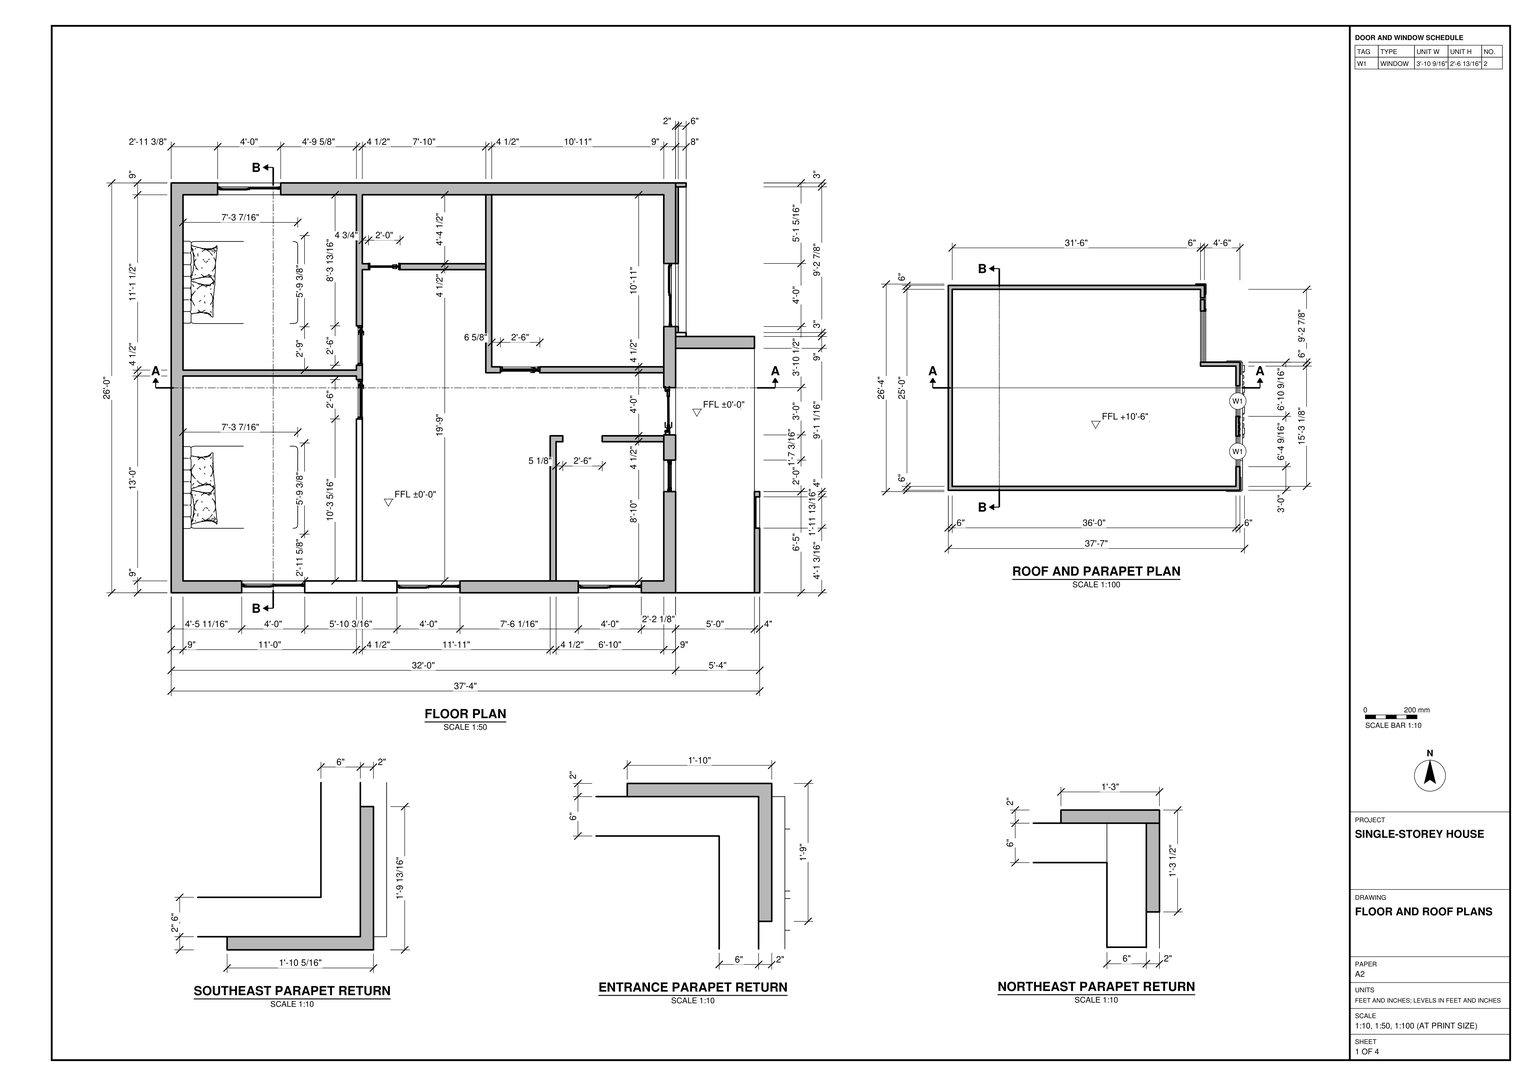
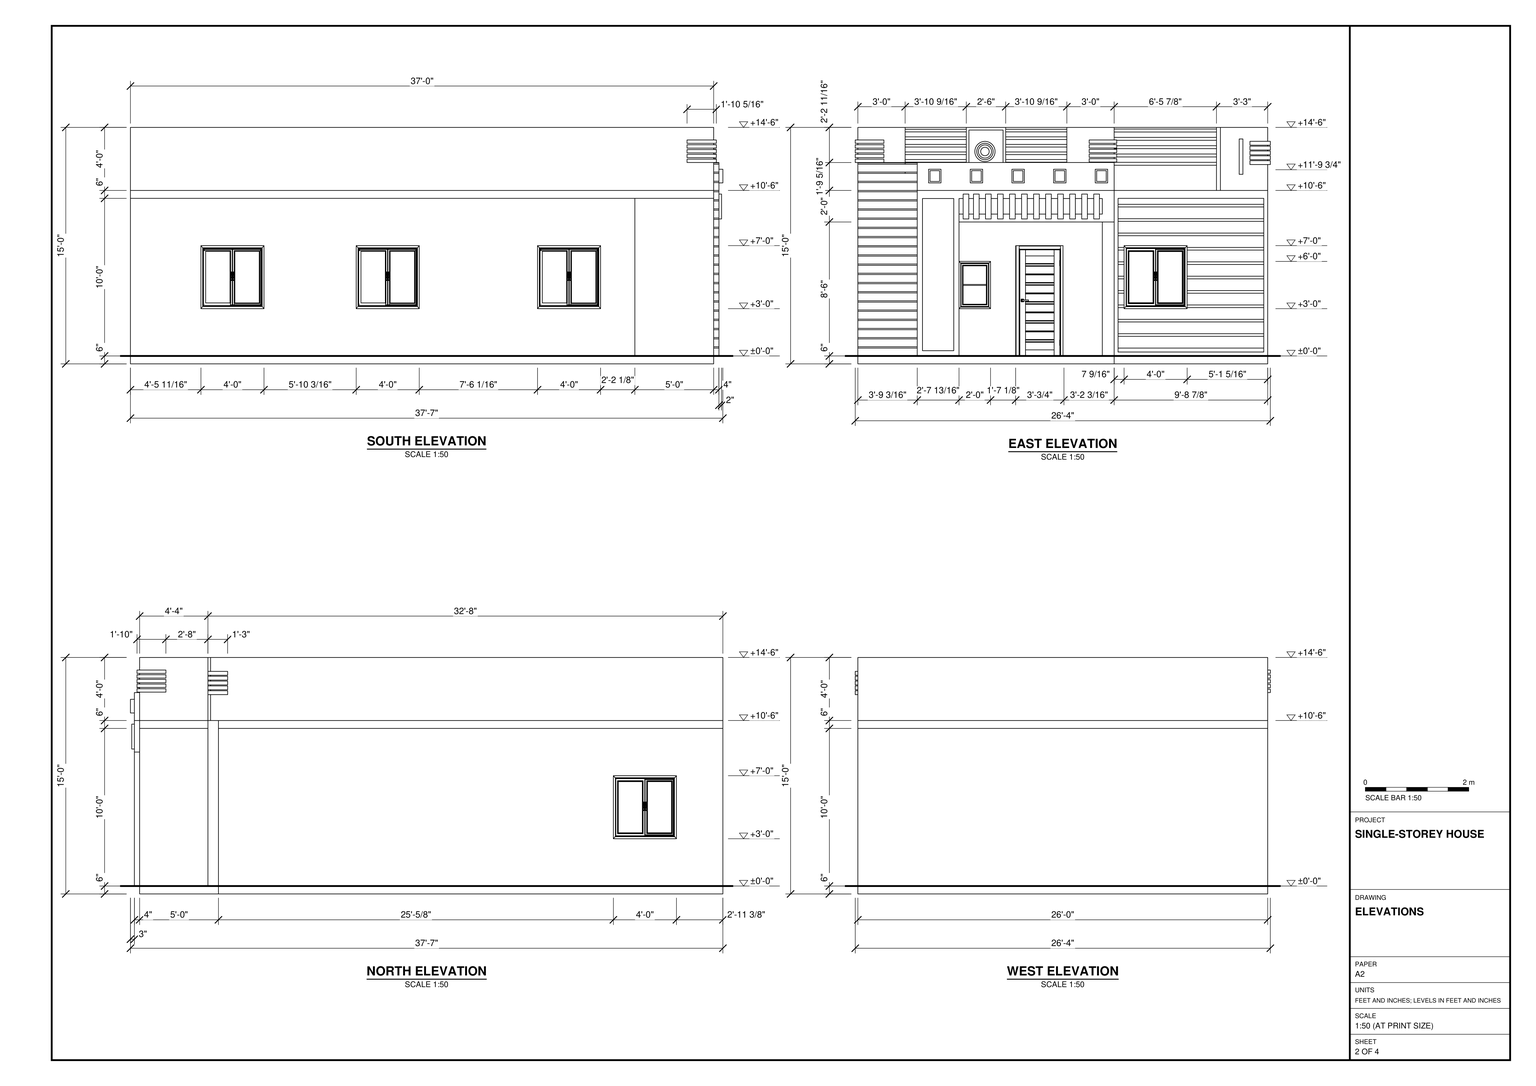
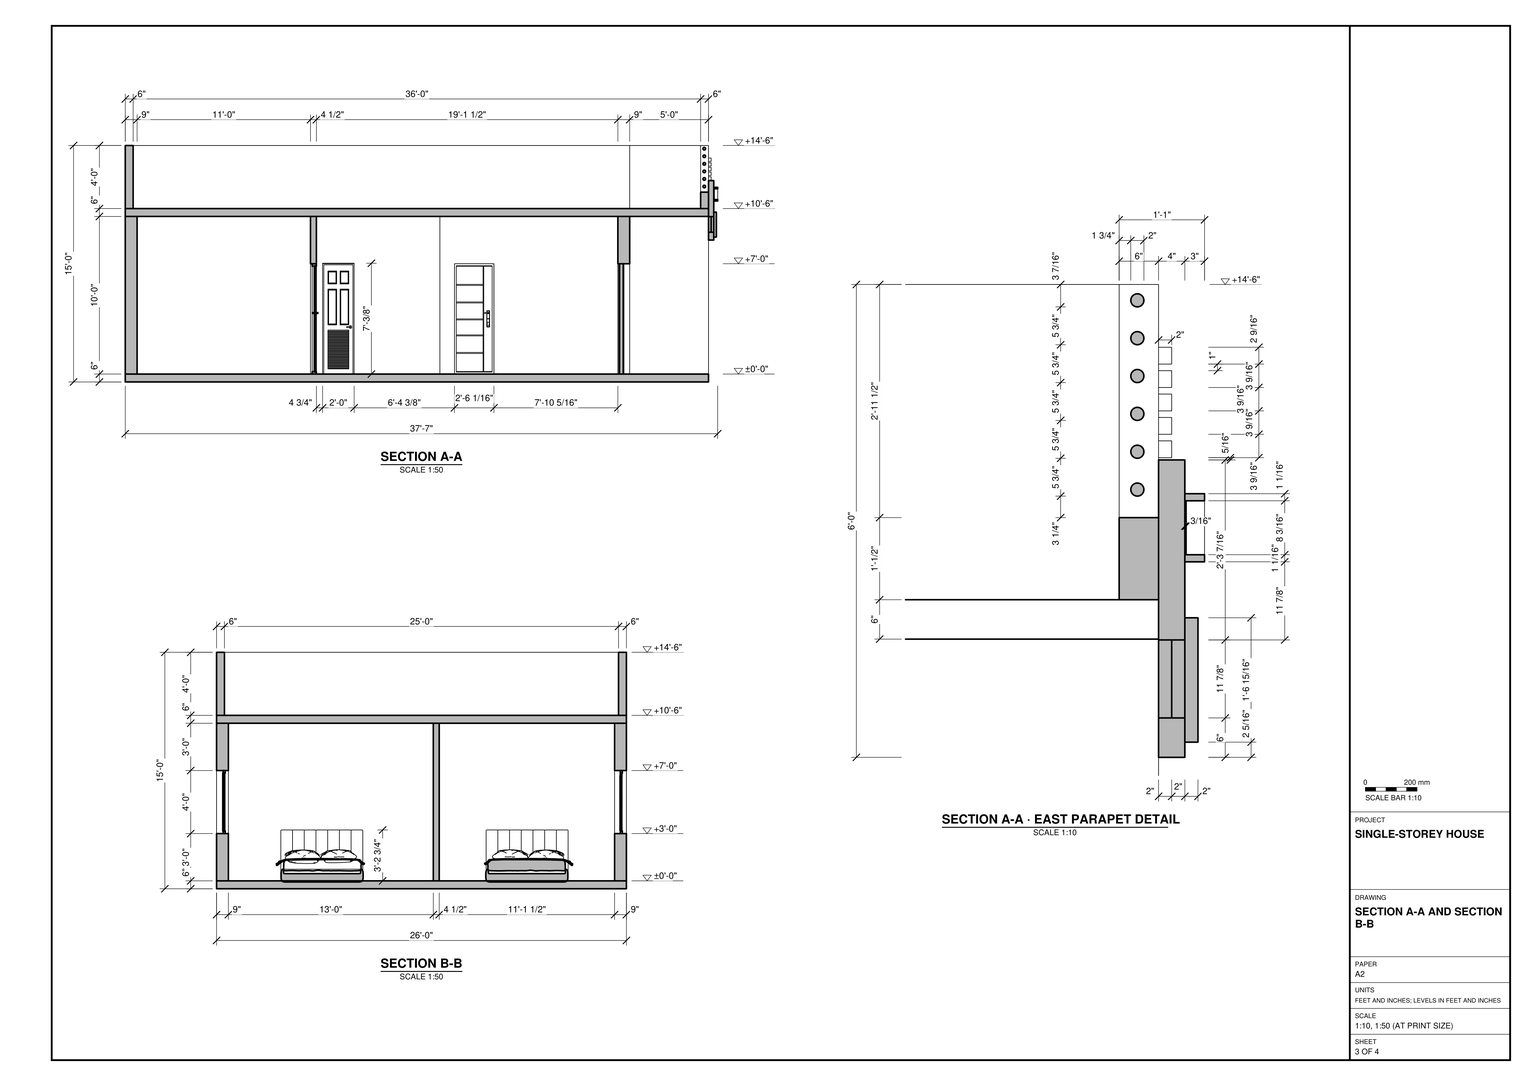
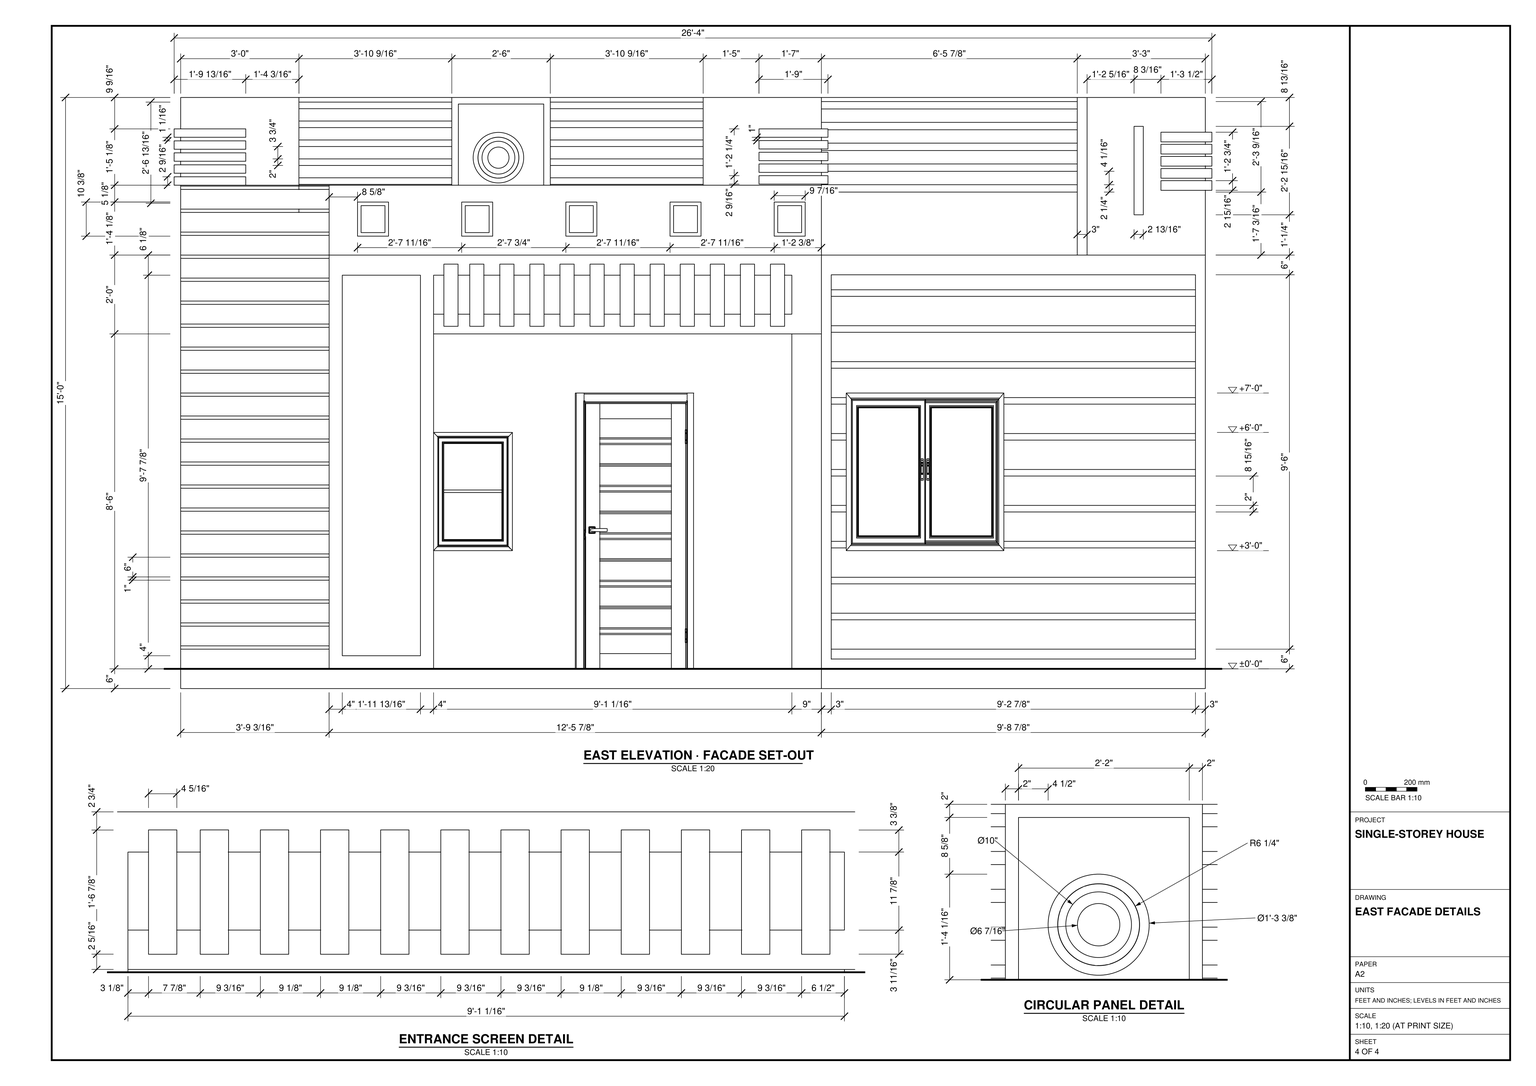
Build the single-storey house in SketchUp using task_files/diagram_01.pdf. Work in feet and inches. Set the finished ground floor at ±0'-0" and model the full exterior, including the slab edges and parapet returns, to an overall size of 37'-7" east to west by 26'-4" north to south by 15'-0" high.

Lay out the main exterior walls at 9" thick and the interior partitions at 4 1/2" thick where indicated. Follow the plan for the two west bedrooms, central circulation space, remaining rooms and covered east entrance. Fit the doors and framed windows in the positions shown. Place a bed against the west wall of each bedroom, matching its footprint in plan and its headboard in section.

Model the floor and flat roof slabs. Set the roof surface at +10'-6" and carry the parapet around the stepped roof outline to +14'-6". Use the east elevation and parapet details to shape the horizontal bands, entrance surround and corner returns; keep the other elevations plain where shown. Decor and loose items may be any suitable library components.

Keep walls, slabs, roof and individual furniture or joinery pieces in separate groups or components, and use components for repeated parts. Save one SketchUp model as output_files/single_storey_house_with_a_recessed_east_entrance.skp.

# SketchUp Ruby script. Lengths in inches.
U = 1.inch
M = Sketchup.active_model
def pt(a) = Geom::Point3d.new(a.map { |v| v * U })
def face(e, loops, mat)
  f = e.add_face(loops[0].map { |a| pt(a) })
  loops[1..].each { |l| e.add_face(l.map { |a| pt(a) }).erase! }
  f.material = f.back_material = mat if mat
  f
end
# faces: each face lists its corners as indices into pts; further lists are holes
def faces(e, pts, list, mat = nil) = list.each { |f| face(e, (f[0].is_a?(Array) ? f : [f]).map { |l| l.map { |i| pts[i] } }, mat) }
# xy, xz, yz: faces in a plane at the given z, y or x. An outline is a flat list of corners, or four numbers for a rectangle; further outlines are holes
def ring(l) = l.size == 4 ? [[l[0], l[1]], [l[2], l[1]], [l[2], l[3]], [l[0], l[3]]] : l.each_slice(2).to_a
def flat(e, list, mat, &to3) = list.each { |f| face(e, (f[0].is_a?(Array) ? f : [f]).map { |l| ring(l).map { |u, v| to3.(u, v) } }, mat) }
def xy(e, z, list, mat = nil) = flat(e, list, mat) { |x, y| [x, y, z] }
def xz(e, y, list, mat = nil) = flat(e, list, mat) { |x, z| [x, y, z] }
def yz(e, x, list, mat = nil) = flat(e, list, mat) { |y, z| [x, y, z] }
def lines(e, pts, list) = list.each { |a, b| e.add_line(pt(pts[a]), pt(pts[b])) }
# prism: a flat outline (further loops are holes) pulled along v
def prism(e, loops, v, mat = nil)
  f = face(e, loops, mat); d = Geom::Vector3d.new(v.map { |x| x * U })
  f.pushpull(f.normal.samedirection?(d) ? d.length : -d.length)
end
def box(e, o, s, mat = nil) = prism(e, [[o, [o[0] + s[0], o[1], o[2]], [o[0] + s[0], o[1] + s[1], o[2]], [o[0], o[1] + s[1], o[2]]]], [0, 0, s[2]], mat)
def at(x, y, z, deg = 0) = Geom::Transformation.translation(pt([x, y, z])) * Geom::Transformation.rotation(ORIGIN, Z_AXIS, deg.degrees)
def axes(o, x, y, z) = Geom::Transformation.new([*x, 0, *y, 0, *z, 0, *pt(o).to_a, 1])
def part(name) = M.definitions.add(name)
# library, detail: a bought-in or finely detailed component or shape, given as its bounding box
def library(name, o, s) = part(name).tap { |d| box(d.entities, o, s) }
def detail(e, o, s) = box(e.add_group.entities, o, s)
def put(e, d, t, mat = nil) = e.add_instance(d, t).tap { |i| i.material = mat if mat }
def group(e, t, mat = nil) = e.add_group.tap { |g| g.transformation = t; g.material = mat if mat }.entities
root = M.entities
M.materials.add("[0003_DeepPink]").color = [255, 20, 147]
M.materials.add("[0005_LightPink]").color = [255, 182, 193]
M.materials.add("[0057_DarkKhaki]").color = [189, 183, 107]
M.materials.add("[0080_DarkCyan]").color = [0, 139, 139]
M.materials.add("[0100_SteelBlue]").color = [70, 130, 180]
M.materials.add("[0109_DarkSlateBlue]").color = [72, 61, 139]
M.materials.add("[0110_LightSlateGray]").color = [119, 136, 153]
M.materials.add("[0127_Magenta]").color = [255, 0, 255]
M.materials.add("[Color A08]").color = [51, 51, 51]
M.materials.add("[Color B07]").color = [153, 38, 0]
M.materials.add("[Color F06]").color = [102, 204, 0]
M.materials.add("[Color H03]").color = [101, 255, 255]
M.materials.add("[Color J07]").color = [76, 0, 153]
M.materials.add("[Color M03]3").color = [132, 147, 124]
M.materials.add("[Color M06]1").color = [61, 61, 61]
M.materials.add("[Field Rectangle Tile]").color = [196, 189, 179]
M.materials.add("[Metal_Corrogated_Shiny]13").color = [12, 12, 12]
M.materials.add("[Metal_Corrogated_Shiny]6").color = [193, 193, 193]
M.materials.add("[Translucent Glass Gray]").color = [128, 128, 128]
c1 = part("Doorknob_Lever_Utility")
xy(c1.entities,0,[[-0.625,-1.08,-1.25,0,-0.625,1.08,0.625,1.08,1.25,0,0.625,-1.08]])
xy(c1.entities,0.25,[[[-0.625,-1.08,0.625,-1.08,1.25,0,0.625,1.08,-0.625,1.08,-1.25,0],[-0.19,-0.33,-0.38,0,-0.19,0.33,0.19,0.33,0.38,0,0.19,-0.33]]])
xy(c1.entities,1.9375,[[-0.19,-0.33,0.19,-0.33,0.38,0,0.19,0.33,-0.19,0.33]])
xz(c1.entities,-1.08,[[-0.625,0,0.625,0.25]])
xz(c1.entities,-0.33,[[-0.19,0.25,0.19,0.25,0.19,1.9375,-0.19,1.9375,-1.49,1.92,-2.79,1.8,-2.75,1.55,-1.48,1.67,-0.19,1.6875]])
xz(c1.entities,0.33,[[-0.19,0.25,-0.19,1.6875,-1.48,1.67,-2.75,1.55,-2.79,1.8,-1.49,1.92,-0.19,1.9375,0.19,1.9375,0.19,0.25]])
xz(c1.entities,1.08,[[-0.625,0,0.625,0.25]])
p = [[-1.25,0,0],[-0.625,-1.08,0],[-0.625,-1.08,0.25],[-1.25,0,0.25],[0.625,-1.08,0],[1.25,0,0],
  [1.25,0,0.25],[0.625,-1.08,0.25],[-0.625,1.08,0],[-0.625,1.08,0.25],[0.625,1.08,0],[0.625,1.08,0.25],
  [-0.19,-0.33,0.25],[-0.19,-0.33,1.6875],[-0.38,0,1.69],[-0.38,0,0.25],[0.19,-0.33,0.25],[0.38,0,0.25],
  [0.38,0,1.9375],[0.19,-0.33,1.9375],[-0.19,0.33,1.6875],[-0.19,0.33,0.25],[0.19,0.33,0.25],[0.19,0.33,1.9375],
  [-4.02,-0.21,1.32],[-2.75,-0.33,1.55],[-4.07,-0.21,1.5625],[-4.02,0.21,1.32],[-2.75,0.33,1.55],[-4.07,0.21,1.5625],
  [-2.79,-0.33,1.8],[-1.48,0.33,1.67],[-1.48,-0.33,1.67],[-2.79,0.33,1.8],[-1.49,-0.33,1.92],[-1.49,0.33,1.92],
  [-0.19,-0.33,1.9375],[-0.19,0.33,1.9375]]
faces(c1.entities,p,[[0,1,2,3],[4,5,6,7],[8,0,3,9],[5,10,11,6],[12,13,14,15],[16,17,18,19],[15,14,20,21],[17,22,23,18],
  [24,25,26],[27,28,25,24],[24,26,29,27],[27,29,28],[30,26,25],[28,31,32,25],[33,28,29],[26,30,33,29],
  [13,32,31,20,14],[33,30,34,35],[36,37,35,34]])
c2 = part("群組\#205")
prism(c2.entities,[[[6.69,3.9375,84.37],[6.69,3.9375,0],[6.69,5.12,0],[6.69,5.12,83.1875],[6.69,34.25,83.1875],[6.69,34.25,0],[6.69,35.43,0],[6.69,35.43,84.37]]],[-7.3,0,0])
c3 = part("群組\#206")
xy(c3.entities,0,[[0,0,1.18,29.13]])
xy(c3.entities,3.95,[[-0.12,4.16,0,24.97],[1.18,4.16,1.3,24.97]])
xy(c3.entities,4.07,[[-0.12,4.28,1.3,24.85]])
xy(c3.entities,33.36,[[-0.12,4.28,1.3,24.85]])
xy(c3.entities,33.48,[[-0.12,4.16,0,24.97],[1.18,4.16,1.3,24.97]])
xy(c3.entities,83.1875,[[0,0,1.18,29.13]])
xz(c3.entities,0,[[0,0,1.18,83.1875]])
xz(c3.entities,4.16,[[-0.12,3.95,0,33.48],[1.18,3.95,1.3,33.48]])
xz(c3.entities,4.28,[[-0.12,4.07,1.3,33.36]])
xz(c3.entities,24.85,[[-0.12,4.07,1.3,33.36]])
xz(c3.entities,24.97,[[-0.12,3.95,0,33.48],[1.18,3.95,1.3,33.48]])
xz(c3.entities,29.13,[[0,0,1.18,83.1875]])
yz(c3.entities,-0.12,[[[4.16,3.95,24.97,33.48],[4.28,4.07,24.85,33.36]]])
yz(c3.entities,0,[[[0,0,29.13,83.1875],[4.16,3.95,24.97,33.48],[16.3,37.41,24.97,64.69],[4.16,37.41,12.83,64.69],[16.3,68.62,24.97,78.46],[4.16,68.62,12.83,78.46]],[4.86,38.2,12.14,63.9],[16.99,38.2,24.28,63.9],[4.86,69.41,12.14,77.68],[16.99,69.41,24.28,77.68]])
yz(c3.entities,0.12,[[[4.27,37.53,12.73,64.57],[4.75,38.08,12.24,64.02]],[[16.41,37.53,24.87,64.57],[16.89,38.08,24.38,64.02]],[[4.27,68.74,12.73,78.35],[4.75,69.29,12.24,77.8]],[[16.41,68.74,24.87,78.35],[16.89,69.29,24.38,77.8]]])
yz(c3.entities,1.0625,[[[4.27,37.53,12.73,64.57],[4.75,38.08,12.24,64.02]],[[16.41,37.53,24.87,64.57],[16.89,38.08,24.38,64.02]],[[4.27,68.74,12.73,78.35],[4.75,69.29,12.24,77.8]],[[16.41,68.74,24.87,78.35],[16.89,69.29,24.38,77.8]]])
yz(c3.entities,1.18,[[[0,0,29.13,83.1875],[4.16,3.95,24.97,33.48],[4.16,37.41,12.83,64.69],[16.3,37.41,24.97,64.69],[4.16,68.62,12.83,78.46],[16.3,68.62,24.97,78.46]],[4.86,38.2,12.14,63.9],[16.99,38.2,24.28,63.9],[4.86,69.41,12.14,77.68],[16.99,69.41,24.28,77.68]])
yz(c3.entities,1.3,[[[4.16,3.95,24.97,33.48],[4.28,4.07,24.85,33.36]]])
p = [[0,4.16,37.41],[0,4.16,64.69],[0.12,4.27,64.57],[0.12,4.27,37.53],[0,12.83,37.41],[0.12,12.73,37.53],
  [1.18,4.16,64.69],[1.18,4.16,37.41],[1.0625,4.27,37.53],[1.0625,4.27,64.57],[1.18,12.83,37.41],[1.0625,12.73,37.53],
  [0,12.83,64.69],[0.12,12.73,64.57],[1.18,12.83,64.69],[1.0625,12.73,64.57],[0,16.3,37.41],[0,16.3,64.69],
  [0.12,16.41,64.57],[0.12,16.41,37.53],[0,24.97,37.41],[0.12,24.87,37.53],[1.18,16.3,64.69],[1.18,16.3,37.41],
  [1.0625,16.41,37.53],[1.0625,16.41,64.57],[1.18,24.97,37.41],[1.0625,24.87,37.53],[0,24.97,64.69],[0.12,24.87,64.57],
  [1.18,24.97,64.69],[1.0625,24.87,64.57],[0.12,4.75,38.08],[0.12,4.75,64.02],[0,4.86,63.9],[0,4.86,38.2],
  [0.12,12.24,38.08],[0,12.14,38.2],[1.0625,4.75,64.02],[1.0625,4.75,38.08],[1.18,4.86,38.2],[1.18,4.86,63.9],
  [1.0625,12.24,38.08],[1.18,12.14,38.2],[0.12,12.24,64.02],[0,12.14,63.9],[1.0625,12.24,64.02],[1.18,12.14,63.9],
  [0.12,24.38,38.08],[0.12,16.89,38.08],[0,16.99,38.2],[0,24.28,38.2],[0.12,16.89,64.02],[0,16.99,63.9],
  [1.0625,16.89,38.08],[1.0625,24.38,38.08],[1.18,24.28,38.2],[1.18,16.99,38.2],[1.0625,16.89,64.02],[1.18,16.99,63.9],
  [0.12,24.38,64.02],[0,24.28,63.9],[1.0625,24.38,64.02],[1.18,24.28,63.9],[0,12.83,68.62],[0,4.16,68.62],
  [0.12,4.27,68.74],[0.12,12.73,68.74],[0,4.16,78.46],[0.12,4.27,78.35],[1.18,4.16,68.62],[1.18,12.83,68.62],
  [1.0625,12.73,68.74],[1.0625,4.27,68.74],[1.18,4.16,78.46],[1.0625,4.27,78.35],[0,12.83,78.46],[0.12,12.73,78.35],
  [1.18,12.83,78.46],[1.0625,12.73,78.35],[0,24.97,68.62],[0,16.3,68.62],[0.12,16.41,68.74],[0.12,24.87,68.74],
  [0,16.3,78.46],[0.12,16.41,78.35],[1.18,16.3,78.46],[1.18,16.3,68.62],[1.0625,16.41,68.74],[1.0625,16.41,78.35],
  [1.18,24.97,68.62],[1.0625,24.87,68.74],[0,24.97,78.46],[0.12,24.87,78.35],[1.18,24.97,78.46],[1.0625,24.87,78.35],
  [0.12,4.75,69.29],[0.12,4.75,77.8],[0,4.86,77.68],[0,4.86,69.41],[0.12,12.24,69.29],[0,12.14,69.41],
  [1.0625,4.75,69.29],[1.0625,12.24,69.29],[1.18,12.14,69.41],[1.18,4.86,69.41],[1.0625,4.75,77.8],[1.18,4.86,77.68],
  [0.12,12.24,77.8],[0,12.14,77.68],[1.0625,12.24,77.8],[1.18,12.14,77.68],[0.12,24.38,69.29],[0.12,16.89,69.29],
  [0,16.99,69.41],[0,24.28,69.41],[0.12,16.89,77.8],[0,16.99,77.68],[1.0625,16.89,69.29],[1.0625,24.38,69.29],
  [1.18,24.28,69.41],[1.18,16.99,69.41],[1.0625,16.89,77.8],[1.18,16.99,77.68],[0.12,24.38,77.8],[0,24.28,77.68],
  [1.0625,24.38,77.8],[1.18,24.28,77.68]]
faces(c3.entities,p,[[0,1,2,3],[4,0,3,5],[6,7,8,9],[7,10,11,8],[12,4,5,13],[10,14,15,11],[16,17,18,19],[20,16,19,21],
  [22,23,24,25],[23,26,27,24],[28,20,21,29],[26,30,31,27],[32,33,34,35],[36,32,35,37],[38,39,40,41],[39,42,43,40],
  [44,36,37,45],[42,46,47,43],[48,49,50,51],[49,52,53,50],[54,55,56,57],[58,54,57,59],[60,48,51,61],[55,62,63,56],
  [33,44,45,34],[46,38,41,47],[52,60,61,53],[62,58,59,63],[1,12,13,2],[14,6,9,15],[17,28,29,18],[30,22,25,31],
  [64,65,66,67],[65,68,69,66],[70,71,72,73],[74,70,73,75],[76,64,67,77],[71,78,79,72],[80,81,82,83],[81,84,85,82],
  [86,87,88,89],[87,90,91,88],[92,80,83,93],[90,94,95,91],[96,97,98,99],[100,96,99,101],[102,103,104,105],[106,102,105,107],
  [108,100,101,109],[103,110,111,104],[112,113,114,115],[113,116,117,114],[118,119,120,121],[122,118,121,123],[124,112,115,125],[119,126,127,120],
  [97,108,109,98],[110,106,107,111],[116,124,125,117],[126,122,123,127],[68,76,77,69],[78,74,75,79],[84,92,93,85],[94,86,89,95]])
c4 = part("群組\#217")
prism(c4.entities,[[[1.42,20.57,0.79],[0,20.57,0],[0,20.57,0.44],[1.42,20.57,1.23]]],[0,-20.57,0])
c5 = part("群組\#207")
put(c5.entities,c1,axes([3.54,31.85,35.81],[0,1,0],[0,0,1],[1,0,0]))
put(c5.entities,c1,axes([2.36,31.85,35.81],[0,1,0],[0,0,-1],[-1,0,0]))
put(c5.entities,c2,at(0,0,0))
put(c5.entities,c3,at(2.36,5.12,0))
put(c5.entities,c4,axes([2.24,9.4,4.07],[1,0,0],[0,1,0],[0,0,0.99041]))
put(c5.entities,c4,axes([2.24,9.4,5.24],[1,0,0],[0,1,0],[0,0,0.99041]))
put(c5.entities,c4,axes([2.24,9.4,6.41],[1,0,0],[0,1,0],[0,0,0.99041]))
put(c5.entities,c4,axes([2.24,9.4,7.58],[1,0,0],[0,1,0],[0,0,0.99041]))
put(c5.entities,c4,axes([2.24,9.4,8.75],[1,0,0],[0,1,0],[0,0,0.99041]))
put(c5.entities,c4,axes([2.24,9.4,9.92],[1,0,0],[0,1,0],[0,0,0.99041]))
put(c5.entities,c4,axes([2.24,9.4,11.09],[1,0,0],[0,1,0],[0,0,0.99041]))
put(c5.entities,c4,axes([2.24,9.4,12.26],[1,0,0],[0,1,0],[0,0,0.99041]))
put(c5.entities,c4,axes([2.24,9.4,13.42],[1,0,0],[0,1,0],[0,0,0.99041]))
put(c5.entities,c4,axes([2.24,9.4,14.59],[1,0,0],[0,1,0],[0,0,0.99041]))
put(c5.entities,c4,axes([2.24,9.4,15.76],[1,0,0],[0,1,0],[0,0,0.99041]))
put(c5.entities,c4,axes([2.24,9.4,16.93],[1,0,0],[0,1,0],[0,0,0.99041]))
put(c5.entities,c4,axes([2.24,9.4,18.1],[1,0,0],[0,1,0],[0,0,0.99041]))
put(c5.entities,c4,axes([2.24,9.4,19.27],[1,0,0],[0,1,0],[0,0,0.99041]))
put(c5.entities,c4,axes([2.24,9.4,20.44],[1,0,0],[0,1,0],[0,0,0.99041]))
put(c5.entities,c4,axes([2.24,9.4,21.61],[1,0,0],[0,1,0],[0,0,0.99041]))
put(c5.entities,c4,axes([2.24,9.4,22.78],[1,0,0],[0,1,0],[0,0,0.99041]))
put(c5.entities,c4,axes([2.24,9.4,23.95],[1,0,0],[0,1,0],[0,0,0.99041]))
put(c5.entities,c4,axes([2.24,9.4,25.12],[1,0,0],[0,1,0],[0,0,0.99041]))
put(c5.entities,c4,axes([2.24,9.4,26.29],[1,0,0],[0,1,0],[0,0,0.99041]))
put(c5.entities,c4,axes([2.24,9.4,27.46],[1,0,0],[0,1,0],[0,0,0.99041]))
put(c5.entities,c4,axes([2.24,9.4,28.63],[1,0,0],[0,1,0],[0,0,0.99041]))
put(c5.entities,c4,axes([2.24,9.4,29.8],[1,0,0],[0,1,0],[0,0,0.99041]))
put(c5.entities,c4,axes([2.24,9.4,30.97],[1,0,0],[0,1,0],[0,0,0.99041]))
put(c5.entities,c4,axes([2.24,9.4,32.14],[1,0,0],[0,1,0],[0,0,0.99041]))
c6 = part("Component")
put(c6.entities,c5,axes([266.12,209.42,0],[0,0.64706,0],[0.762,0,0],[0,0,1]))
c7 = library("BED 3",[-244.73,-59.6875,196.6875],[91.01,69.4,39.64])
c8 = part("Component\#10")
xy(c8.entities,0,[[20,0,20,19,0,19,0,21,22,21,22,0]])
xy(c8.entities,2.5625,[[20,0,22,0,22,21,0,21,0,19,20,19]])
xz(c8.entities,0,[[20,0,22,2.5625]])
xz(c8.entities,21,[[0,0,22,2.5625]])
yz(c8.entities,0,[[19,0,21,2.5625]])
yz(c8.entities,20,[[0,0,19,2.5625]])
yz(c8.entities,22,[[0,0,21,2.5625]])
c9 = part("Component\#3")
xy(c9.entities,0,[[0,0,3,9.4375]],"[0100_SteelBlue]")
xy(c9.entities,1.08,[[0,1.08,0.1875,8.36],[0.1875,1.08,3,8.36]],"[0100_SteelBlue]")
xy(c9.entities,9.29,[[0,1.08,0.1875,8.36],[0.1875,1.08,3,8.36]],"[0100_SteelBlue]")
xy(c9.entities,10.375,[[0,0,3,9.4375]],"[0100_SteelBlue]")
xz(c9.entities,0,[[0,0,3,10.375]],"[0100_SteelBlue]")
xz(c9.entities,1.08,[[0,1.08,0.1875,9.29],[0.1875,1.08,3,9.29]],"[0100_SteelBlue]")
xz(c9.entities,8.36,[[0,1.08,0.1875,9.29],[0.1875,1.08,3,9.29]],"[0100_SteelBlue]")
xz(c9.entities,9.4375,[[0,0,3,10.375]],"[0100_SteelBlue]")
yz(c9.entities,0,[[[0,0,9.4375,10.375],[1.08,1.08,8.36,9.29]]],"[0100_SteelBlue]")
yz(c9.entities,0.1875,[[1.08,1.08,8.36,9.29]],"[Color F06]")
yz(c9.entities,3,[[[0,0,9.4375,10.375],[1.08,1.08,8.36,9.29]]],"[0100_SteelBlue]")
c10 = part("Component\#4")
box(c10.entities,[2.75,0,0],[18.9375,4.3125,2],"[Color B07]")
c11 = library("mesh-166",[-1553.69,-2604.3125,-42.18],[1702.88,1401.6,88.28])
c12 = part("Group17")
put(c12.entities,c11,at(294.66,859.51,3.5))
c13 = library("mesh-158",[272.88,-1887.9,-41.96],[1017.57,1401.85,65.81])
c14 = part("Component\#74")
xy(c14.entities,0,[[0,1.57,11.02,2.98]])
xy(c14.entities,5.07,[[4.05,-4.05,4.95,-1.24],[4.95,-4.05,5.6,-1.24],[5.6,-4.05,5.6,-1.24,6.76,-1.24,6.76,-2.48,18.91,-2.48,18.91,-4.05],[4.4375,-1.24,4.95,0.17],[4.95,-1.24,5.6,0.17],
  [5.6,-1.24,6.76,0.17]],"[Metal_Corrogated_Shiny]13")
xy(c14.entities,7.43,[[4.05,-4.05,18.91,-4.05,18.91,-2.48,6.76,-2.48,6.76,-1.24,4.05,-1.24],[4.4375,-1.24,6.76,0.17]],"[Metal_Corrogated_Shiny]13")
xy(c14.entities,44.08,[[0,1.57,11.02,2.98]],"[Metal_Corrogated_Shiny]13")
xz(c14.entities,-4.05,[[4.05,5.07,18.91,7.43]],"[Metal_Corrogated_Shiny]13")
xz(c14.entities,-2.48,[[6.76,5.07,18.91,7.43]],"[Metal_Corrogated_Shiny]13")
xz(c14.entities,-1.24,[[4.05,5.07,4.4375,7.43],[4.4375,5.07,6.76,7.43]],"[Metal_Corrogated_Shiny]13")
xz(c14.entities,0.17,[[[5.87,3.92,6.43,4.04,6.9375,4.32,7.36,4.72,7.67,5.22,7.84,5.78,7.86,6.375,7.73,6.95,7.47,7.47,7.08,7.91,6.59,8.22,6.05,8.4,5.47,8.42,4.91,8.29,4.41,8.02,3.98,7.62,3.68,7.12,3.51,6.55,3.48,5.96,3.61,5.39,3.875,4.87,4.27,4.43,4.75,4.12,5.3,3.9375],[4.4375,5.07,6.76,7.43]]],"[Metal_Corrogated_Shiny]13")
xz(c14.entities,1.57,[[1.9,30.99,8.98,39.82]])
xz(c14.entities,1.57,[[[1.125,22.3125,10.125,42.95],[1.9,30.99,8.98,39.82]]],"[Metal_Corrogated_Shiny]13")
xz(c14.entities,1.57,[[[0,0,11.02,44.08],[1.125,22.3125,10.125,42.95],[1.125,1.125,10.125,21.3125]],[[1.125,1.125,10.125,21.3125],[5.87,3.92,5.3,3.9375,4.75,4.12,4.27,4.43,3.875,4.87,3.61,5.39,3.48,5.96,3.51,6.55,3.68,7.12,3.98,7.62,4.41,8.02,4.91,8.29,5.47,8.42,6.05,8.4,6.59,8.22,7.08,7.91,7.47,7.47,7.73,6.95,7.86,6.375,7.84,5.78,7.67,5.22,7.36,4.72,6.9375,4.32,6.43,4.04]]],"[Metal_Corrogated_Shiny]6")
xz(c14.entities,2.98,[[0,0,11.02,44.08]])
yz(c14.entities,0,[[1.57,0,2.98,44.08]],"[Metal_Corrogated_Shiny]13")
yz(c14.entities,4.05,[[-4.05,5.07,-1.24,7.43]],"[Metal_Corrogated_Shiny]13")
yz(c14.entities,4.4375,[[-1.24,5.07,0.17,7.43]],"[Metal_Corrogated_Shiny]13")
yz(c14.entities,6.76,[[-2.48,5.07,-1.24,7.43],[-1.24,5.07,0.17,7.43]],"[Metal_Corrogated_Shiny]13")
yz(c14.entities,11.02,[[1.57,0,2.98,44.08]],"[Metal_Corrogated_Shiny]13")
yz(c14.entities,18.91,[[-4.05,5.07,-2.48,7.43]],"[Metal_Corrogated_Shiny]13")
# 6 loose lines left out
p = [[4.75,1.57,4.12],[5.3,1.57,3.9375],[5.3,0.17,3.9375],[4.75,0.17,4.12],[5.87,1.57,3.92],[5.87,0.17,3.92],
  [6.43,1.57,4.04],[6.43,0.17,4.04],[6.9375,1.57,4.32],[6.9375,0.17,4.32],[4.27,1.57,4.43],[4.27,0.17,4.43],
  [7.36,1.57,4.72],[7.36,0.17,4.72],[3.875,1.57,4.87],[3.875,0.17,4.87],[7.67,1.57,5.22],[7.67,0.17,5.22],
  [3.61,1.57,5.39],[3.61,0.17,5.39],[7.84,1.57,5.78],[7.84,0.17,5.78],[3.48,1.57,5.96],[3.48,0.17,5.96],
  [7.86,1.57,6.375],[7.86,0.17,6.375],[3.51,1.57,6.55],[3.51,0.17,6.55],[7.73,1.57,6.95],[7.73,0.17,6.95],
  [3.68,1.57,7.12],[3.68,0.17,7.12],[7.47,1.57,7.47],[7.47,0.17,7.47],[3.98,1.57,7.62],[3.98,0.17,7.62],
  [7.08,1.57,7.91],[7.08,0.17,7.91],[4.41,1.57,8.02],[4.41,0.17,8.02],[6.59,1.57,8.22],[6.59,0.17,8.22],
  [4.91,1.57,8.29],[4.91,0.17,8.29],[6.05,1.57,8.4],[6.05,0.17,8.4],[5.47,1.57,8.42],[5.47,0.17,8.42]]
faces(c14.entities,p,[[0,1,2,3],[1,4,5,2],[4,6,7,5],[6,8,9,7],[10,0,3,11],[8,12,13,9],[14,10,11,15],[12,16,17,13],
  [18,14,15,19],[16,20,21,17],[22,18,19,23],[20,24,25,21],[26,22,23,27],[24,28,29,25],[30,26,27,31],[28,32,33,29],
  [34,30,31,35],[32,36,37,33],[38,34,35,39],[36,40,41,37],[42,38,39,43],[40,44,45,41],[46,42,43,47],[44,46,47,45]],"[Metal_Corrogated_Shiny]13")
c15 = part("建立群組\#163")
prism(c15.entities,[[[3.9375,61.02,0],[3.9375,61.02,86.61],[3.9375,17.71,86.61],[3.9375,17.71,0]],[[3.9375,19.68,84.65],[3.9375,59.06,84.65],[3.9375,59.06,1.97],[3.9375,19.68,1.97]]],[-3.9375,0,0])
c16 = part("建立群組\#165")
xy(c16.entities,0,[[0,0,39.375,1.57]])
xy(c16.entities,83.46,[[0,0,39.375,1.57]])
xz(c16.entities,0,[[0,0,29.375,14.65],[30.16,0,39.375,83.46],[0,15.43,29.375,28.43],[0,29.21,29.375,41.73],[0,42.52,29.375,54.29],
  [0,55.08,29.375,68.07],[0,68.86,29.375,83.46]])
xz(c16.entities,0,[[29.375,0,30.16,83.46],[0,14.65,29.375,15.43],[0,28.43,29.375,29.21],[0,41.73,29.375,42.52],[0,54.29,29.375,55.08],
  [0,68.07,29.375,68.86]],"[Color A08]")
xz(c16.entities,1.57,[[0,0,23.35,83.46],[24.14,0,30.33,61.79],[31.12,0,39.375,83.46],[24.14,61.79,30.33,83.46]])
xz(c16.entities,1.57,[[23.35,0,24.14,83.46],[30.33,0,31.12,83.46]],"[Color M03]3")
yz(c16.entities,0,[[0,0,1.57,83.46]])
yz(c16.entities,39.375,[[0,0,1.57,83.46]])
c17 = part("建立群組\#164")
put(c17.entities,c16,at(-25.45,-11.17,1.57))
c18 = part("建立群組\#166")
put(c18.entities,c14,axes([2.72,21.88,36.87],[0,0.29138,0],[-0.2535,0,0],[0,0,0.29138]))
put(c18.entities,c14,axes([-0.36,22.42,36.87],[0,0.29138,0],[0.2535,0,0],[0,0,0.29138]))
put(c18.entities,c15,at(0,0,0),"[Color M06]1")
put(c18.entities,c17,at(11.57,33.6,0,-90),"[Color M06]1")
c19 = library("Группа\#16",[0,0,0],[5.38,37.87,81.85])
c20 = library("Group\#19",[-438,-2,0],[446,316,48])
xy(root,0,[[384,186.1,444,195.1]],"[0109_DarkSlateBlue]")
xy(root,0,[[444,0,448,77.01]],"[Color J07]")
xy(root,4,[[445,49.2,448,73.01]],"[0127_Magenta]")
xy(root,6,[[444,0,448,45.2]],"[Color J07]")
xy(root,7,[[444,0,448,45.2]])
xy(root,13,[[444,0,448,45.2]],"[Color J07]")
xy(root,14,[[444,0,448,45.2]])
xy(root,20,[[444,0,448,45.2]],"[Color J07]")
xy(root,21,[[444,0,448,45.2]])
xy(root,27,[[444,0,448,45.2]],"[Color J07]")
xy(root,28,[[444,0,448,45.2]])
xy(root,34,[[444,0,448,45.2]],"[Color J07]")
xy(root,35,[[444,0,448,45.2]],"[Color J07]")
xy(root,41,[[444,0,448,45.2]],"[Color J07]")
xy(root,42,[[444,0,448,45.2]],"[Color J07]")
xy(root,48,[[444,0,448,45.2]],"[Color J07]")
xy(root,49,[[444,0,448,45.2]],"[Color J07]")
xy(root,55,[[444,0,448,45.2]],"[Color J07]")
xy(root,56,[[444,0,448,45.2]],"[Color J07]")
xy(root,62,[[444,0,448,45.2]],"[Color J07]")
xy(root,63,[[444,0,448,45.2]],"[Color J07]")
xy(root,69,[[444,0,448,45.2]],"[Color J07]")
xy(root,70,[[444,0,448,45.2]],"[Color J07]")
xy(root,76,[[444,0,448,45.2]],"[Color J07]")
xy(root,77,[[444,0,448,45.2]],"[Color J07]")
xy(root,83,[[444,0,448,45.2]],"[Color J07]")
xy(root,84,[[444,0,448,45.2]],"[Color J07]")
xy(root,90,[[444,0,448,45.2]],"[Color J07]")
xy(root,91,[[444,0,448,45.2]],"[Color J07]")
xy(root,97,[[444,0,448,45.2]],"[Color J07]")
xy(root,98,[[444,0,448,45.2]],"[Color J07]")
xy(root,102,[[444,77.01,448,195.1]],"[0127_Magenta]")
xy(root,104,[[444,0,448,45.2]],"[Color J07]")
xy(root,105,[[444,0,448,45.2]],"[Color J07]")
xy(root,108,[[444,77.01,446,186.1],[446,77.01,448,186.1]],"[0127_Magenta]")
xy(root,111,[[444,0,448,45.2]],"[Color J07]")
xy(root,112,[[444,0,448,45.2]],"[Color J07]")
xy(root,118,[[444,0,448,45.2]],"[Color J07]")
xy(root,119,[[444,0,448,45.2]],"[Color J07]")
xy(root,119.875,[[445,49.2,448,73.01],[444,77.01,446,186.1],[446,77.01,448,186.1]],"[0127_Magenta]")
xy(root,120,[[384,186.1,444,195.1]],"[0109_DarkSlateBlue]")
xy(root,125,[[444,0,448,45.2]],"[Color J07]")
xy(root,126,[[444,0,448,45.2]],"[Color J07]")
xy(root,132,[[444,0,448,45.2]],"[Color J07]")
xy(root,133,[[444,0,448,45.2]],"[Color J07]")
xy(root,139,[[444,0,448,45.2]],"[Color J07]")
xy(root,140,[[444,0,448,45.2]],"[Color J07]")
xy(root,146,[[444,0,448,45.2]],"[Color J07]")
xy(root,147,[[444,0,448,45.2]])
xy(root,147.28,[[444,0,448,195.1]],"[Color J07]")
xz(root,0,[[444,0,448,6],[444,7,448,13],[444,14,448,20],[444,21,448,27],[444,28,448,34],
  [444,35,448,41],[444,42,448,48],[444,49,448,55],[444,56,448,62],[444,63,448,69],
  [444,70,448,76],[444,77,448,83],[444,84,448,90],[444,91,448,97],[444,98,448,104],
  [444,105,448,111],[444,112,448,118],[444,119,448,125],[444,126,448,132],[444,133,448,139],
  [444,140,448,146],[444,147,448,147.28]],"[Color J07]")
xz(root,0,[[384,0,444,120]],"[Translucent Glass Gray]")
xz(root,45.2,[[444,6,448,7],[444,13,448,14],[444,20,448,21],[444,27,448,28],[444,34,448,35],
  [444,41,448,42],[444,48,448,49],[444,55,448,56],[444,62,448,63],[444,69,448,70],
  [444,76,448,77],[444,83,448,84],[444,90,448,91],[444,97,448,98],[444,104,448,105],
  [444,111,448,112],[444,118,448,119],[444,125,448,126],[444,132,448,133],[444,139,448,140],
  [444,146,448,147]])
xz(root,49.2,[[445,4,448,119.875]],"[0127_Magenta]")
xz(root,73.01,[[445,4,448,119.875]],"[0127_Magenta]")
xz(root,77.01,[[444,0,448,102],[444,102,448,108],[444,108,446,119.875],[446,108,448,119.875]],"[0127_Magenta]")
xz(root,186.1,[[384,0,444,120]],"[0110_LightSlateGray]")
xz(root,186.1,[[446,108,448,119.875]],"[0127_Magenta]")
xz(root,195.1,[[444,126,448,147.28]])
xz(root,195.1,[[384,0,438,120],[438,0,444,120]],"[0110_LightSlateGray]")
xz(root,195.1,[[444,102,448,126]],"[0127_Magenta]")
yz(root,384,[[186.1,0,195.1,120]],"[0109_DarkSlateBlue]")
yz(root,444,[[0,0,0,6,45.2,6,45.2,7,0,7,0,13,45.2,13,45.2,14,0,14,0,20,45.2,20,45.2,21,0,21,0,27,45.2,27,45.2,28,0,28,0,34,45.2,34,45.2,35,0,35,0,41,45.2,41,45.2,42,0,42,0,48,45.2,48,45.2,49,0,49,0,55,45.2,55,45.2,56,0,56,0,62,45.2,62,45.2,63,0,63,0,69,45.2,69,45.2,70,0,70,0,76,45.2,76,45.2,77,0,77,0,83,45.2,83,45.2,84,0,84,0,90,45.2,90,45.2,91,0,91,0,97,45.2,97,45.2,98,0,98,0,104,45.2,104,45.2,105,0,105,0,111,45.2,111,45.2,112,0,112,0,118,45.2,118,45.2,119,0,119,0,125,45.2,125,45.2,126,0,126,0,132,45.2,132,45.2,133,0,133,0,139,45.2,139,45.2,140,0,140,0,146,45.2,146,45.2,147,0,147,0,147.28,195.1,147.28,195.1,120,186.1,120,186.1,119.875,77.01,119.875,77.01,0],[0,6,45.2,7],[0,13,45.2,14],[0,20,45.2,21],[0,27,45.2,28],
  [0,34,45.2,35],[0,41,45.2,42],[0,48,45.2,49],[0,55,45.2,56],[0,62,45.2,63],
  [0,69,45.2,70],[0,76,45.2,77],[0,83,45.2,84],[0,97,45.2,98],[0,104,45.2,105],
  [0,111,45.2,112],[0,118,45.2,119]])
yz(root,444,[[186.1,102,195.1,120]],"[0109_DarkSlateBlue]")
yz(root,444,[[186.1,0,195.1,102]],"[0110_LightSlateGray]")
yz(root,444,[[77.01,102,186.1,108],[77.01,108,186.1,119.875]],"[0127_Magenta]")
yz(root,444,[[0,90,45.2,91]],"[Color J07]")
yz(root,445,[[49.2,4,73.01,119.875]],"[0080_DarkCyan]")
yz(root,446,[[77.01,108,186.1,119.875]],"[0110_LightSlateGray]")
yz(root,448,[[[45.2,0,77.01,0,77.01,102,195.1,102,195.1,126,45.2,126],[49.2,4,73.01,119.875],[77.01,108,186.1,119.875]]],"[0127_Magenta]")
yz(root,448,[[0,0,45.2,6],[0,7,45.2,13],[0,14,45.2,20],[0,21,45.2,27],[0,28,45.2,34],
  [0,35,45.2,41],[0,42,45.2,48],[0,49,45.2,55],[0,56,45.2,62],[0,63,45.2,69],
  [0,70,45.2,76],[0,77,45.2,83],[0,84,45.2,90],[0,91,45.2,97],[0,98,45.2,104],
  [0,105,45.2,111],[0,112,45.2,118],[0,119,45.2,125],[0,126,45.2,132],[0,133,45.2,139],
  [0,140,45.2,146],[0,147,45.2,147.28]],"[Color J07]")
put(root,c6,at(-118.89,36.97,0))
put(root,c7,at(250.03,104.31,-197.57))
put(root,c7,axes([250.03,212.22,-197.57],[1,0,0],[0,-1,0],[0,0,1]))
put(root,c8,at(424,176.1,161.875),"[0127_Magenta]")
put(root,c8,at(424,176.1,158.3125),"[0127_Magenta]")
put(root,c8,at(424,176.1,154.75),"[0127_Magenta]")
put(root,c8,at(424,176.1,151.1875),"[0127_Magenta]")
put(root,c8,at(424,176.1,147.625),"[0127_Magenta]")
put(root,c9,at(448,53.85,131.77))
put(root,c9,at(448,85.57,131.77))
put(root,c9,at(448,117.28,131.77))
put(root,c9,at(448,149,131.77))
put(root,c9,at(448,180.72,131.77))
put(root,c10,axes([448,88.02,126],[0,0,-1],[0,1,0],[1,0,0]))
put(root,c10,axes([448,97.17,126],[0,0,-1],[0,1,0],[1,0,0]))
put(root,c10,axes([448,106.33,126],[0,0,-1],[0,1,0],[1,0,0]))
put(root,c10,axes([448,115.49,126],[0,0,-1],[0,1,0],[1,0,0]))
put(root,c10,axes([448,124.64,126],[0,0,-1],[0,1,0],[1,0,0]))
put(root,c10,axes([448,133.8,126],[0,0,-1],[0,1,0],[1,0,0]))
put(root,c10,axes([448,142.95,126],[0,0,-1],[0,1,0],[1,0,0]))
put(root,c10,axes([448,152.11,126],[0,0,-1],[0,1,0],[1,0,0]))
put(root,c10,axes([448,161.27,126],[0,0,-1],[0,1,0],[1,0,0]))
put(root,c10,axes([448,170.42,126],[0,0,-1],[0,1,0],[1,0,0]))
put(root,c10,axes([448,179.58,126],[0,0,-1],[0,1,0],[1,0,0]))
put(root,c10,axes([448,80.14,126],[0,0,-1],[0,1,0],[1,0,0]))
put(root,c12,axes([379.64,238.15,95.75],[0,0.02819,0],[0,0,0.03425],[0.02402,0,0]))
g1 = group(root,at(378.71,88.96,54))
put(g1,c13,axes([0.38,-18.39,30.49],[0,0.02359,0],[0,0,0.02568],[-0.03937,0,0]))
put(root,c12,axes([322.41,4.55,95.75],[-0.02819,0,0],[0,0,0.03425],[0,0.02402,0]))
put(root,c12,axes([184.375,4.55,95.75],[-0.02819,0,0],[0,0,0.03425],[0,0.02402,0]))
put(root,c12,axes([66.17,5.43,95.75],[-0.02819,0,0],[0,0,0.03425],[0,0.02402,0]))
put(root,c12,axes([47.87,307.75,95.75],[-0.02819,0,0],[0,0,0.03425],[0,0.02402,0]))
put(root,c18,axes([292.96,168.63,84],[0,0.81344,0],[-0.69372,0,0],[0,0,-0.96982]))
put(root,c18,axes([145.5,174.62,84],[-0.81344,0,0],[0,-0.69372,0],[0,0,-0.96982]))
put(root,c18,axes([145.5,215.51,84],[-0.81344,0,0],[0,-0.69372,0],[0,0,-0.96982]))
put(root,c19,axes([381.06,156.9,0],[-0.99999,-0.00519,0],[0.00503,-0.96999,0],[0,0,1.02626]))
g2 = group(root,at(0,0,120),"[Color J07]")
prism(g2,[[[0,312,0],[384,312,0],[384,195.1,0],[444,195.1,0],[444,0,0],[0,0,0]]],[0,0,6],"[0057_DarkKhaki]")
g3 = group(root,at(0,0,-6))
xy(g3,0,[[0,0,0,312,384,312,384,195.1,444,195.1,444,0]],"[0057_DarkKhaki]")
xy(g3,6,[[0,0,444,0,444,195.1,384,195.1,384,312,0,312]],"[Field Rectangle Tile]")
xz(g3,0,[[0,0,444,6]],"[0057_DarkKhaki]")
xz(g3,195.1,[[384,0,444,6]],"[0057_DarkKhaki]")
xz(g3,312,[[0,0,384,6]],"[0057_DarkKhaki]")
yz(g3,0,[[0,0,312,6]],"[0057_DarkKhaki]")
yz(g3,384,[[195.1,0,312,6]],"[0057_DarkKhaki]")
yz(g3,444,[[0,0,195.1,6]],"[0057_DarkKhaki]")
g4 = group(root,at(0,0,0))
xy(g4,0,[[0,0,0,312,384,312,384,156.17,375,156.17,375,303,9,303,9,9,375,9,375,120.17,384,120.17,384,0],[288.5,9,288.5,119.5,298.1,119.5,298.1,115,293,115,293,9],[328.1,115,375,119.5],[239.5,167.5,239.5,303,244,303,244,172,250.625,172,250.625,167.5],[280.625,167.5,375,172]],"[0005_LightPink]")
xy(g4,36,[[53.66,0,101.66,9],[171.87,0,219.87,9],[309.9,0,357.9,9],[375,77.01,384,101.01],[375,202.66,384,250.66],
  [35.36,303,83.36,312]],"[0005_LightPink]")
xy(g4,72,[[375,77.01,384,101.01]],"[0005_LightPink]")
xy(g4,84,[[53.66,0,101.66,9],[171.87,0,219.87,9],[309.9,0,357.9,9],[298.1,115,328.1,119.5],[375,120.17,384,156.17],
  [141,132.29,145.5,162.29],[250.625,167.5,280.625,172],[141,173.18,145.5,203.18],[375,202.66,384,250.66],[150.23,246,174.23,250.5],
  [35.36,303,83.36,312]],"[0005_LightPink]")
xy(g4,120,[[[0,0,384,312],[9,9,375,303]],[141,9,145.5,9,145.5,303,141,303,141,169.5,9,169.5,9,165,141,165],[288.5,9,293,9,293,115,375,115,375,119.5,288.5,119.5],[239.5,167.5,375,167.5,375,172,244,172,244,303,239.5,303],[145.5,246,239.5,250.5]],"[0005_LightPink]")
xz(g4,0,[[[0,0,384,120],[309.9,36,357.9,84],[171.87,36,219.87,84],[53.66,36,101.66,84]]],"[0005_LightPink]")
xz(g4,9,[[[9,0,141,120],[53.66,36,101.66,84]],[[145.5,0,288.5,120],[171.87,36,219.87,84]],[288.5,0,293,120],[[293,0,375,120],[309.9,36,357.9,84]]],"[0005_LightPink]")
xz(g4,77.01,[[375,36,384,72]],"[0005_LightPink]")
xz(g4,101.01,[[375,36,384,72]],"[0005_LightPink]")
xz(g4,115,[[293,0,298.1,0,298.1,84,328.1,84,328.1,0,375,0,375,120,293,120]],"[0005_LightPink]")
xz(g4,119.5,[[288.5,0,288.5,120,375,120,375,0,328.1,0,328.1,84,298.1,84,298.1,0]],"[0005_LightPink]")
xz(g4,120.17,[[375,0,384,84]],"[0005_LightPink]")
xz(g4,132.29,[[141,0,145.5,84]],"[0005_LightPink]")
xz(g4,156.17,[[375,0,384,84]],"[0005_LightPink]")
xz(g4,162.29,[[141,0,145.5,84]],"[0005_LightPink]")
xz(g4,165,[[9,0,141,120]],"[0005_LightPink]")
xz(g4,167.5,[[239.5,0,250.625,0,250.625,84,280.625,84,280.625,0,375,0,375,120,239.5,120]],"[0005_LightPink]")
xz(g4,169.5,[[9,0,141,120]],"[0005_LightPink]")
xz(g4,172,[[244,0,244,120,375,120,375,0,280.625,0,280.625,84,250.625,84,250.625,0]],"[0005_LightPink]")
xz(g4,173.18,[[141,0,145.5,84]],"[0005_LightPink]")
xz(g4,202.66,[[375,36,384,84]],"[0005_LightPink]")
xz(g4,203.18,[[141,0,145.5,84]],"[0005_LightPink]")
xz(g4,246,[[145.5,0,150.23,0,150.23,84,174.23,84,174.23,0,239.5,0,239.5,120,145.5,120]],"[0005_LightPink]")
xz(g4,250.5,[[145.5,0,145.5,120,239.5,120,239.5,0,174.23,0,174.23,84,150.23,84,150.23,0]],"[0005_LightPink]")
xz(g4,250.66,[[375,36,384,84]],"[0005_LightPink]")
xz(g4,303,[[[9,0,141,120],[35.36,36,83.36,84]],[145.5,0,239.5,120],[239.5,0,244,120],[244,0,375,120]],"[0005_LightPink]")
xz(g4,312,[[[0,0,384,120],[35.36,36,83.36,84]]],"[0005_LightPink]")
yz(g4,0,[[0,0,312,120]],"[0005_LightPink]")
yz(g4,9,[[9,0,165,120],[169.5,0,303,120]],"[0005_LightPink]")
yz(g4,35.36,[[303,36,312,84]],"[0005_LightPink]")
yz(g4,53.66,[[0,36,9,84]],"[0005_LightPink]")
yz(g4,83.36,[[303,36,312,84]],"[0005_LightPink]")
yz(g4,101.66,[[0,36,9,84]],"[0005_LightPink]")
yz(g4,141,[[9,0,9,120,165,120,165,0,162.29,0,162.29,84,132.29,84,132.29,0],[169.5,0,169.5,120,303,120,303,0,203.18,0,203.18,84,173.18,84,173.18,0]],"[0005_LightPink]")
yz(g4,145.5,[[9,0,132.29,0,132.29,84,162.29,84,162.29,0,173.18,0,173.18,84,203.18,84,203.18,0,246,0,246,120,9,120],[250.5,0,303,120]],"[0005_LightPink]")
yz(g4,150.23,[[246,0,250.5,84]],"[0005_LightPink]")
yz(g4,171.87,[[0,36,9,84]],"[0005_LightPink]")
yz(g4,174.23,[[246,0,250.5,84]],"[0005_LightPink]")
yz(g4,219.87,[[0,36,9,84]],"[0005_LightPink]")
yz(g4,239.5,[[167.5,0,246,120],[246,0,250.5,120],[250.5,0,303,120]],"[0005_LightPink]")
yz(g4,244,[[172,0,303,120]],"[0005_LightPink]")
yz(g4,250.625,[[167.5,0,172,84]],"[0005_LightPink]")
yz(g4,280.625,[[167.5,0,172,84]],"[0005_LightPink]")
yz(g4,288.5,[[9,0,119.5,120]],"[0005_LightPink]")
yz(g4,293,[[9,0,115,120]],"[0005_LightPink]")
yz(g4,298.1,[[115,0,119.5,84]],"[0005_LightPink]")
yz(g4,309.9,[[0,36,9,84]],"[0005_LightPink]")
yz(g4,328.1,[[115,0,119.5,84]],"[0005_LightPink]")
yz(g4,357.9,[[0,36,9,84]],"[0005_LightPink]")
yz(g4,375,[[[9,0,115,120],[77.01,36,101.01,72]],[115,0,119.5,120],[119.5,0,119.5,120,167.5,120,167.5,0,156.17,0,156.17,84,120.17,84,120.17,0],[167.5,0,172,120],[[172,0,303,120],[202.66,36,250.66,84]]],"[0005_LightPink]")
yz(g4,384,[[[0,0,120.17,0,120.17,84,156.17,84,156.17,0,198.1,0,198.1,120,0,120],[77.01,36,101.01,72]],[[198.1,0,312,120],[202.66,36,250.66,84]]],"[0005_LightPink]")
# 1 loose lines left out
g5 = group(root,at(384,198.1,0),"[0003_DeepPink]")
box(g5,[0,0,115.4375],[2,110.9,4.5625])
prism(g5,[[[2,110.9,27.89],[2,110.9,36.83],[2,52.5625,36.83],[2,52.5625,36],[2,4.5625,36],[2,4.5625,36.83],[2,0,36.83],[2,0,27.89]]],[-2,0,0])
prism(g5,[[[2,110.9,82.61],[2,110.9,91.55],[2,0,91.55],[2,0,82.61],[2,4.5625,82.61],[2,4.5625,84],[2,52.5625,84],[2,52.5625,82.61]]],[-2,0,0])
box(g5,[0,0,6],[2,110.9,8.94])
box(g5,[0,0,38.83],[2,4.5625,8.95])
box(g5,[0,0,60.72],[2,4.5625,8.94])
box(g5,[0,0,71.66],[2,4.5625,8.95])
box(g5,[0,0,16.94],[2,110.9,8.95])
box(g5,[0,52.5625,38.83],[2,58.34,8.95])
box(g5,[0,52.5625,49.78],[2,58.34,8.94])
box(g5,[0,52.5625,60.72],[2,58.34,8.94])
box(g5,[0,52.5625,71.66],[2,58.34,8.95])
box(g5,[0,0,93.55],[2,110.9,8.94])
box(g5,[0,0,104.49],[2,110.9,8.95])
box(g5,[0,0,49.78],[2,4.5625,8.94])
g6 = group(root,at(384,195.1,-6),"[Color H03]")
prism(g6,[[[8,0,6],[8,116.9,6],[8,116.9,132],[8,0,132]],[[8,3,126],[8,113.9,126],[8,113.9,9],[8,3,9]]],[-8,0,0])
# 1 loose lines left out
put(root,c20,at(438,0,126))
g7 = group(root,at(448,45.2,126))
yz(g7,0,[[0,0,149.9,21.28]])
